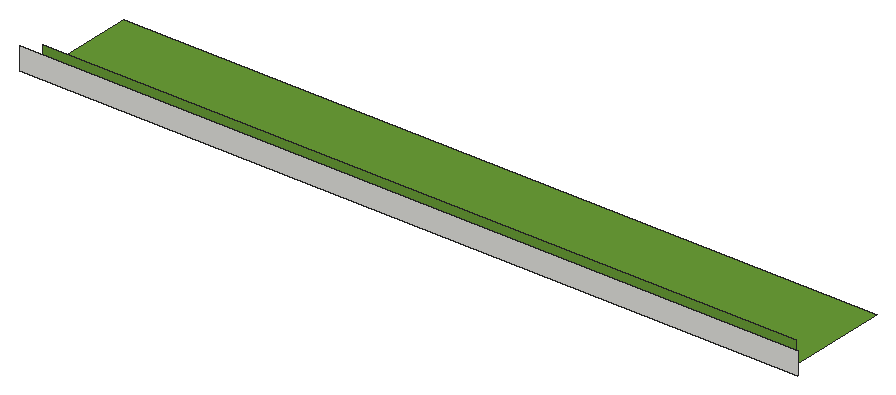
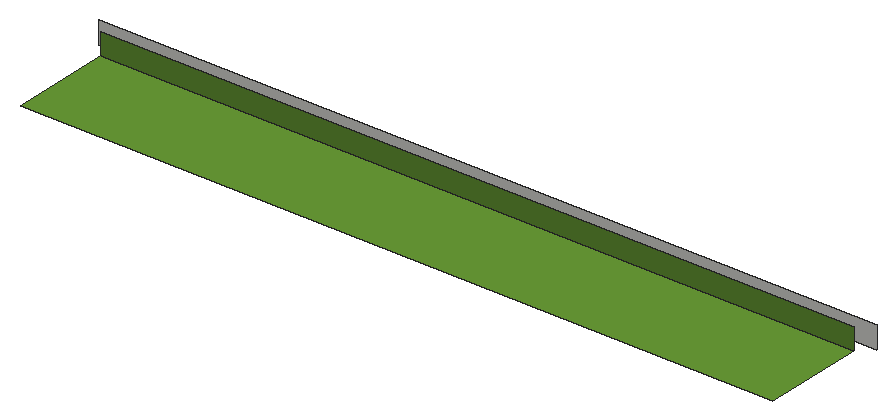
# SketchUp Ruby script. Lengths in inches.
U = 1.inch
M = Sketchup.active_model
def pt(a) = Geom::Point3d.new(a.map { |v| v * U })
def face(e, loops, mat)
  f = e.add_face(loops[0].map { |a| pt(a) })
  loops[1..].each { |l| e.add_face(l.map { |a| pt(a) }).erase! }
  f.material = f.back_material = mat if mat
  f
end
# faces: each face lists its corners as indices into pts; further lists are holes
def faces(e, pts, list, mat = nil) = list.each { |f| face(e, (f[0].is_a?(Array) ? f : [f]).map { |l| l.map { |i| pts[i] } }, mat) }
# xy, xz, yz: faces in a plane at the given z, y or x. An outline is a flat list of corners, or four numbers for a rectangle; further outlines are holes
def ring(l) = l.size == 4 ? [[l[0], l[1]], [l[2], l[1]], [l[2], l[3]], [l[0], l[3]]] : l.each_slice(2).to_a
def flat(e, list, mat, &to3) = list.each { |f| face(e, (f[0].is_a?(Array) ? f : [f]).map { |l| ring(l).map { |u, v| to3.(u, v) } }, mat) }
def xy(e, z, list, mat = nil) = flat(e, list, mat) { |x, y| [x, y, z] }
def xz(e, y, list, mat = nil) = flat(e, list, mat) { |x, z| [x, y, z] }
def yz(e, x, list, mat = nil) = flat(e, list, mat) { |y, z| [x, y, z] }
def lines(e, pts, list) = list.each { |a, b| e.add_line(pt(pts[a]), pt(pts[b])) }
# prism: a flat outline (further loops are holes) pulled along v
def prism(e, loops, v, mat = nil)
  f = face(e, loops, mat); d = Geom::Vector3d.new(v.map { |x| x * U })
  f.pushpull(f.normal.samedirection?(d) ? d.length : -d.length)
end
def box(e, o, s, mat = nil) = prism(e, [[o, [o[0] + s[0], o[1], o[2]], [o[0] + s[0], o[1] + s[1], o[2]], [o[0], o[1] + s[1], o[2]]]], [0, 0, s[2]], mat)
def at(x, y, z, deg = 0) = Geom::Transformation.translation(pt([x, y, z])) * Geom::Transformation.rotation(ORIGIN, Z_AXIS, deg.degrees)
def axes(o, x, y, z) = Geom::Transformation.new([*x, 0, *y, 0, *z, 0, *pt(o).to_a, 1])
def part(name) = M.definitions.add(name)
# library, detail: a bought-in or finely detailed component or shape, given as its bounding box
def library(name, o, s) = part(name).tap { |d| box(d.entities, o, s) }
def detail(e, o, s) = box(e.add_group.entities, o, s)
def put(e, d, t, mat = nil) = e.add_instance(d, t).tap { |i| i.material = mat if mat }
def group(e, t, mat = nil) = e.add_group.tap { |g| g.transformation = t; g.material = mat if mat }.entities
root = M.entities
M.materials.add("[Grass Dark Green]").color = [106, 157, 55]
xy(root,9,[[25.26,47.13,277.5,80.93]],"[Grass Dark Green]")
xz(root,42.875,[[21.01,9,281.76,16.375]])
xz(root,47.13,[[25.26,9,277.5,16.375]],"[Grass Dark Green]")
